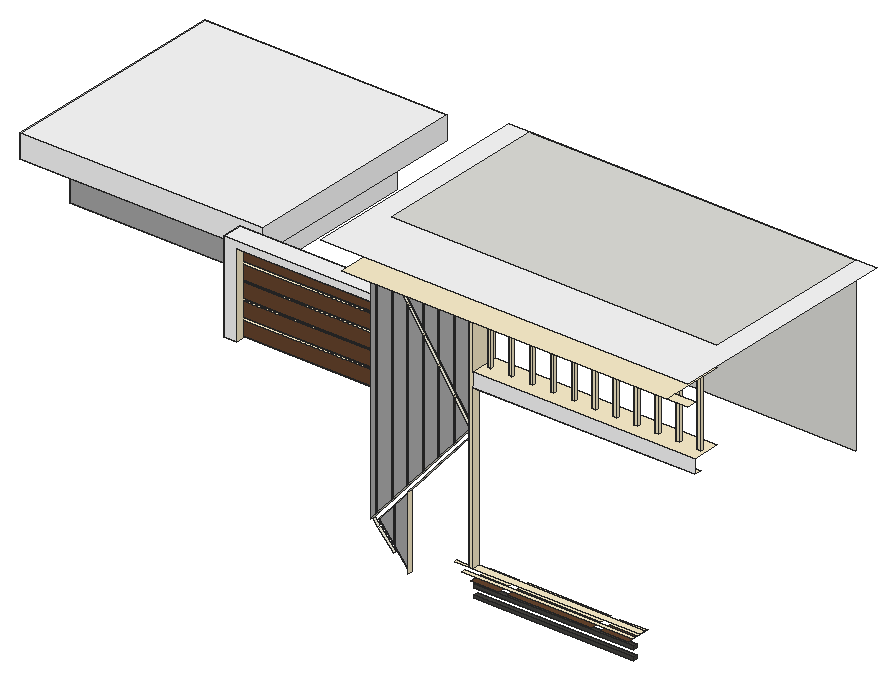
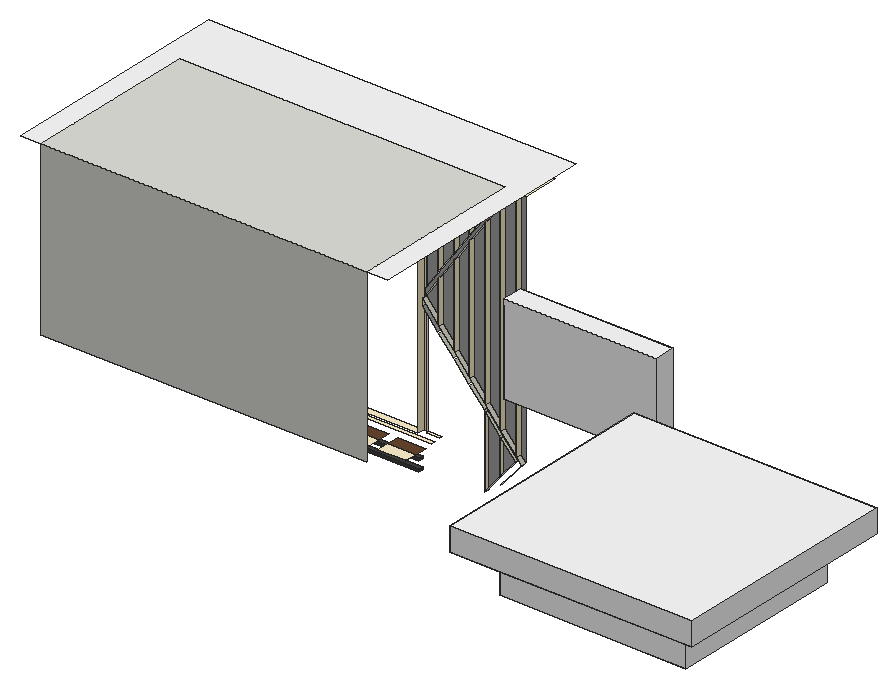
# SketchUp Ruby script. Lengths in inches.
U = 1.inch
M = Sketchup.active_model
def pt(a) = Geom::Point3d.new(a.map { |v| v * U })
def face(e, loops, mat)
  f = e.add_face(loops[0].map { |a| pt(a) })
  loops[1..].each { |l| e.add_face(l.map { |a| pt(a) }).erase! }
  f.material = f.back_material = mat if mat
  f
end
# faces: each face lists its corners as indices into pts; further lists are holes
def faces(e, pts, list, mat = nil) = list.each { |f| face(e, (f[0].is_a?(Array) ? f : [f]).map { |l| l.map { |i| pts[i] } }, mat) }
# xy, xz, yz: faces in a plane at the given z, y or x. An outline is a flat list of corners, or four numbers for a rectangle; further outlines are holes
def ring(l) = l.size == 4 ? [[l[0], l[1]], [l[2], l[1]], [l[2], l[3]], [l[0], l[3]]] : l.each_slice(2).to_a
def flat(e, list, mat, &to3) = list.each { |f| face(e, (f[0].is_a?(Array) ? f : [f]).map { |l| ring(l).map { |u, v| to3.(u, v) } }, mat) }
def xy(e, z, list, mat = nil) = flat(e, list, mat) { |x, y| [x, y, z] }
def xz(e, y, list, mat = nil) = flat(e, list, mat) { |x, z| [x, y, z] }
def yz(e, x, list, mat = nil) = flat(e, list, mat) { |y, z| [x, y, z] }
def lines(e, pts, list) = list.each { |a, b| e.add_line(pt(pts[a]), pt(pts[b])) }
# prism: a flat outline (further loops are holes) pulled along v
def prism(e, loops, v, mat = nil)
  f = face(e, loops, mat); d = Geom::Vector3d.new(v.map { |x| x * U })
  f.pushpull(f.normal.samedirection?(d) ? d.length : -d.length)
end
def box(e, o, s, mat = nil) = prism(e, [[o, [o[0] + s[0], o[1], o[2]], [o[0] + s[0], o[1] + s[1], o[2]], [o[0], o[1] + s[1], o[2]]]], [0, 0, s[2]], mat)
def at(x, y, z, deg = 0) = Geom::Transformation.translation(pt([x, y, z])) * Geom::Transformation.rotation(ORIGIN, Z_AXIS, deg.degrees)
def axes(o, x, y, z) = Geom::Transformation.new([*x, 0, *y, 0, *z, 0, *pt(o).to_a, 1])
def part(name) = M.definitions.add(name)
# library, detail: a bought-in or finely detailed component or shape, given as its bounding box
def library(name, o, s) = part(name).tap { |d| box(d.entities, o, s) }
def detail(e, o, s) = box(e.add_group.entities, o, s)
def put(e, d, t, mat = nil) = e.add_instance(d, t).tap { |i| i.material = mat if mat }
def group(e, t, mat = nil) = e.add_group.tap { |g| g.transformation = t; g.material = mat if mat }.entities
root = M.entities
M.materials.add("D01_Frost_White").color = [255, 242, 206]
M.materials.add("M00_Soft_Cloud").color = [255, 255, 255]
M.materials.add("M03_Pewter_Shine").color = [168, 168, 168]
M.materials.add("Metal_06_1K").color = [238, 236, 219]
M.materials.add("Wood_Planks_01_1K").color = [69, 67, 63]
M.materials.add("Wood_Veneer_15_1K").color = [103, 69, 45]
xy(root,235.08,[[313.01,117.13,382.01,119.15]],"Wood_Planks_01_1K")
xy(root,236.46,[[313.01,117.13,382.01,119.15]],"Wood_Planks_01_1K")
xy(root,239.33,[[313.01,117.13,382.01,119.15]],"Wood_Planks_01_1K")
xy(root,240.7,[[313.01,117.13,382.01,119.15]],"Wood_Planks_01_1K")
xy(root,242.68,[[313.01,115.54,313.02,126],[313.02,120.77,325.01,126],[329.01,120.77,365.01,126],[369.01,120.77,381.02,126]],"D01_Frost_White")
xy(root,242.68,[[313.02,115.54,325.01,120.77],[329.01,115.54,365.01,120.77],[369.01,115.54,381.02,120.77]],"Wood_Veneer_15_1K")
xy(root,245.68,[[310.01,114,384.02,115.54]],"D01_Frost_White")
xy(root,248.68,[[307.01,114,313.02,115],[315.02,114,387.02,117]],"D01_Frost_White")
xy(root,290,[[194.88,129,194.88,138,261.02,138,261.02,133.24,200.88,133.24,200.88,129],[96.73,168.8,177.62,244.72]],"D01_Frost_White")
xy(root,291,[[200.88,132.24,261.02,133.24]],"D01_Frost_White")
xy(root,297.25,[[200.88,132.24,261.02,133.24]],"D01_Frost_White")
xy(root,298.25,[[200.88,132.24,261.02,133.24]],"D01_Frost_White")
xy(root,304.5,[[200.88,132.24,261.02,133.24]],"D01_Frost_White")
xy(root,305.5,[[200.88,132.24,261.02,133.24]],"D01_Frost_White")
xy(root,308,[[96.73,168.8,177.62,244.72]],"D01_Frost_White")
xy(root,308,[[84.73,156.8,189.62,168.8],[84.73,168.8,96.73,256.72],[177.62,168.8,189.62,256.72],[96.73,244.72,177.62,256.72]],"M00_Soft_Cloud")
xy(root,311.75,[[200.88,132.24,261.02,133.24]],"D01_Frost_White")
xy(root,312.75,[[200.88,132.24,261.02,133.24]],"D01_Frost_White")
xy(root,318,[[84.73,156.8,189.62,256.72]],"M00_Soft_Cloud")
xy(root,319,[[315.02,114,387.02,117],[387.02,114,411.02,117],[200.88,132.24,261.02,133.24]],"D01_Frost_White")
xy(root,320,[[200.88,132.24,261.02,133.24]],"D01_Frost_White")
xy(root,325,[[[315.02,114,411.02,126],[316.82,119.67,318.36,120.6875]]],"D01_Frost_White")
xy(root,326,[[200.88,129,261.02,132.24]],"D01_Frost_White")
xy(root,328.95,[[194.88,129,261.02,138]],"M00_Soft_Cloud")
xy(root,355,[[270.02,99,270.02,115,272.24,115,272.24,117,272.74,117,272.74,115,275.84,115,275.84,116,277.34,116,277.34,115,278.95,115,278.95,117,279.45,117,279.45,115,285.67,115,285.67,117,286.17,117,286.17,115,292.38,115,292.38,117,292.88,117,292.88,115,299.09,115,299.09,117,299.59,117,299.59,115,305.81,115,305.81,117,306.31,117,306.31,115,313.02,115,313.02,114,315.02,114,315.02,126,411.02,126,411.02,99],[411.02,99,420.02,103.1]],"D01_Frost_White")
xy(root,356.67,[[316.82,119.67,318.36,120.6875],[325.875,119.67,327.42,120.6875],[334.93,119.67,336.47,120.6875],[343.99,119.67,345.53,120.6875],[353.05,119.67,354.59,120.6875],
  [362.11,119.67,363.65,120.6875],[371.17,119.67,372.71,120.6875],[380.23,119.67,381.77,120.6875],[389.29,119.67,390.83,120.6875],[398.34,119.67,399.88,120.6875],
  [407.4,119.67,408.94,120.6875]],"D01_Frost_White")
xy(root,364,[[270.02,126,411.02,201]])
xy(root,364,[[261.02,99,420.02,99,420.02,201,411.02,201,411.02,126,270.02,126,270.02,201,261.02,201]],"M00_Soft_Cloud")
xz(root,114,[[313.02,248.68,315.02,355]],"D01_Frost_White")
xz(root,114,[[315.02,319,411.02,325]],"M00_Soft_Cloud")
xz(root,115,[[270.02,251.83,272.24,254.41,272.24,355,270.02,355],[272.74,254.99,278.95,262.22,278.95,350.56,275.84,355,272.74,355],[279.45,262.8,285.67,270.02,285.67,340.96,279.45,349.84],[286.17,270.61,292.38,277.83,292.38,331.36,286.17,340.24],[292.88,278.41,299.09,285.64,299.09,321.76,292.88,330.64],
  [299.59,286.22,305.81,293.45,305.81,312.15,299.59,321.04],[306.31,294.03,313.02,301.84,306.31,311.44],[313.02,304.84,313.02,355,306.31,355,306.31,314.28],[305.81,314.98,305.81,355,299.59,355,299.59,323.72],[299.09,324.42,299.09,355,292.88,355,292.88,333.16],
  [292.38,333.86,292.38,355,286.17,355,286.17,342.6],[285.67,343.3,285.67,355,279.45,355,279.45,352.04],[278.95,352.74,278.95,355,277.34,355]],"M03_Pewter_Shine")
xz(root,116,[[285.67,236.55,285.67,267.27,279.45,260.1,279.45,244.15],[278.95,244.76,278.95,259.53,272.74,252.36],[313.02,301.84,313.02,304.84,306.31,314.28,305.81,314.98,299.59,323.72,299.09,324.42,292.88,333.16,292.38,333.86,286.17,342.6,285.67,343.3,279.45,352.04,278.95,352.74,277.34,355,275.84,355,278.95,350.56,279.45,349.84,285.67,340.96,286.17,340.24,292.38,331.36,292.88,330.64,299.09,321.76,299.59,321.04,305.81,312.15,306.31,311.44]],"M03_Pewter_Shine")
xz(root,117,[[286.17,235.93,286.17,267.85,285.67,267.27,285.67,236.55],[279.45,244.15,279.45,260.1,278.95,259.53,278.95,244.76],[272.24,254.41,272.74,254.99,272.74,355,272.24,355],[278.95,262.22,279.45,262.8,279.45,349.84,278.95,350.56],[285.67,270.02,286.17,270.61,286.17,340.24,285.67,340.96],
  [292.38,277.83,292.88,278.41,292.88,330.64,292.38,331.36],[299.09,285.64,299.59,286.22,299.59,321.04,299.09,321.76],[305.81,293.45,306.31,294.03,306.31,311.44,305.81,312.15],[306.31,314.28,306.31,355,305.81,355,305.81,314.98],[299.59,323.72,299.59,355,299.09,355,299.09,324.42],
  [292.88,333.16,292.88,355,292.38,355,292.38,333.86],[286.17,342.6,286.17,355,285.67,355,285.67,343.3],[279.45,352.04,279.45,355,278.95,355,278.95,352.74]],"D01_Frost_White")
xz(root,117.13,[[313.01,235.08,382.01,236.46],[313.01,239.33,382.01,240.7]],"Wood_Planks_01_1K")
xz(root,119.15,[[313.01,235.08,382.01,236.46],[313.01,239.33,382.01,240.7]],"Wood_Planks_01_1K")
xz(root,119.67,[[316.82,325,318.36,356.67],[325.875,325,327.42,356.67],[334.93,325,336.47,356.67],[343.99,325,345.53,356.67],[353.05,325,354.59,356.67],
  [362.11,325,363.65,356.67],[371.17,325,372.71,356.67],[380.23,325,381.77,356.67],[389.29,325,390.83,356.67],[398.34,325,399.88,356.67],
  [407.4,325,408.94,356.67]],"D01_Frost_White")
xz(root,120.6875,[[316.82,325,318.36,356.67],[325.875,325,327.42,356.67],[334.93,325,336.47,356.67],[343.99,325,345.53,356.67],[353.05,325,354.59,356.67],
  [362.11,325,363.65,356.67],[371.17,325,372.71,356.67],[380.23,325,381.77,356.67],[389.29,325,390.83,356.67],[398.34,325,399.88,356.67],
  [407.4,325,408.94,356.67]],"D01_Frost_White")
xz(root,129,[[194.88,290,200.88,290,200.88,326,261.02,326,261.02,328.95,194.88,328.95]],"M00_Soft_Cloud")
xz(root,132.24,[[200.88,291,261.02,297.25],[200.88,298.25,261.02,304.5],[200.88,305.5,261.02,311.75],[200.88,312.75,261.02,319],[200.88,320,261.02,326]],"Wood_Veneer_15_1K")
xz(root,133.24,[[200.88,290,261.02,291],[200.88,297.25,261.02,298.25],[200.88,304.5,261.02,305.5],[200.88,311.75,261.02,312.75],[200.88,319,261.02,320]],"D01_Frost_White")
xz(root,138,[[194.88,290,261.02,328.95]],"M00_Soft_Cloud")
xz(root,156.8,[[84.73,308,189.62,318]],"M00_Soft_Cloud")
xz(root,168.8,[[96.73,290,177.62,308]],"M03_Pewter_Shine")
xz(root,201,[[270.02,290,411.02,364]])
xz(root,244.72,[[96.73,290,177.62,308]],"M00_Soft_Cloud")
xz(root,256.72,[[84.73,308,189.62,318]],"M00_Soft_Cloud")
yz(root,84.73,[[156.8,308,256.72,318]],"M00_Soft_Cloud")
yz(root,96.73,[[168.8,290,244.72,308]],"M00_Soft_Cloud")
yz(root,177.62,[[168.8,290,244.72,308]],"M00_Soft_Cloud")
yz(root,189.62,[[156.8,308,256.72,318]],"M00_Soft_Cloud")
yz(root,194.88,[[129,290,138,328.95]],"M00_Soft_Cloud")
yz(root,200.88,[[129,290,133.24,290,133.24,291,132.24,291,132.24,297.25,133.24,297.25,133.24,298.25,132.24,298.25,132.24,304.5,133.24,304.5,133.24,305.5,132.24,305.5,132.24,311.75,133.24,311.75,133.24,312.75,132.24,312.75,132.24,319,133.24,319,133.24,320,132.24,320,132.24,326,129,326]],"D01_Frost_White")
yz(root,261.02,[[133.24,290,133.24,291,132.24,291,132.24,297.25,133.24,297.25,133.24,298.25,132.24,298.25,132.24,304.5,133.24,304.5,133.24,305.5,132.24,305.5,132.24,311.75,133.24,311.75,133.24,312.75,132.24,312.75,132.24,319,133.24,319,133.24,320,132.24,320,132.24,326,138,326,138,290]],"D01_Frost_White")
yz(root,272.24,[[115,254.41,117,355]],"D01_Frost_White")
yz(root,272.74,[[115,254.99,117,355]],"D01_Frost_White")
yz(root,278.95,[[116,244.76,117,259.53],[115,262.22,117,350.56],[115,352.74,117,355]],"D01_Frost_White")
yz(root,279.45,[[116,244.15,117,260.1],[115,262.8,117,349.84],[115,352.04,117,355]],"D01_Frost_White")
yz(root,285.67,[[116,236.55,117,267.27],[115,270.02,117,340.96],[115,343.3,117,355]],"D01_Frost_White")
yz(root,286.17,[[115,235.93,117,267.85],[115,270.61,117,340.24],[115,342.6,117,355]],"D01_Frost_White")
yz(root,292.38,[[115,277.83,117,331.36],[115,333.86,117,355]],"D01_Frost_White")
yz(root,292.88,[[115,278.41,117,330.64],[115,333.16,117,355]],"D01_Frost_White")
yz(root,299.09,[[115,285.64,117,321.76],[115,324.42,117,355]],"D01_Frost_White")
yz(root,299.59,[[115,286.22,117,321.04],[115,323.72,117,355]],"D01_Frost_White")
yz(root,305.81,[[115,293.45,117,312.15],[115,314.98,117,355]],"D01_Frost_White")
yz(root,306.31,[[115,294.03,117,311.44],[115,314.28,117,355]],"D01_Frost_White")
yz(root,313.02,[[114,248.68,115,298.84],[114,298.84,114,355,115,355,115,304.84,116,304.84,116,301.84,117,301.84,117,298.84]],"D01_Frost_White")
yz(root,315.02,[[114,248.68,117,319],[114,325,126,355]],"D01_Frost_White")
yz(root,316.82,[[119.67,325,120.6875,356.67]],"D01_Frost_White")
yz(root,318.36,[[119.67,325,120.6875,356.67]],"D01_Frost_White")
yz(root,325.875,[[119.67,325,120.6875,356.67]],"D01_Frost_White")
yz(root,327.42,[[119.67,325,120.6875,356.67]],"D01_Frost_White")
yz(root,334.93,[[119.67,325,120.6875,356.67]],"D01_Frost_White")
yz(root,336.47,[[119.67,325,120.6875,356.67]],"D01_Frost_White")
yz(root,343.99,[[119.67,325,120.6875,356.67]],"D01_Frost_White")
yz(root,345.53,[[119.67,325,120.6875,356.67]],"D01_Frost_White")
yz(root,353.05,[[119.67,325,120.6875,356.67]],"D01_Frost_White")
yz(root,354.59,[[119.67,325,120.6875,356.67]],"D01_Frost_White")
yz(root,362.11,[[119.67,325,120.6875,356.67]],"D01_Frost_White")
yz(root,363.65,[[119.67,325,120.6875,356.67]],"D01_Frost_White")
yz(root,371.17,[[119.67,325,120.6875,356.67]],"D01_Frost_White")
yz(root,372.71,[[119.67,325,120.6875,356.67]],"D01_Frost_White")
yz(root,380.23,[[119.67,325,120.6875,356.67]],"D01_Frost_White")
yz(root,381.77,[[119.67,325,120.6875,356.67]],"D01_Frost_White")
yz(root,382.01,[[117.13,235.08,119.15,236.46],[117.13,239.33,119.15,240.7]],"Wood_Planks_01_1K")
yz(root,389.29,[[119.67,325,120.6875,356.67]],"D01_Frost_White")
yz(root,390.83,[[119.67,325,120.6875,356.67]],"D01_Frost_White")
yz(root,398.34,[[119.67,325,120.6875,356.67]],"D01_Frost_White")
yz(root,399.88,[[119.67,325,120.6875,356.67]],"D01_Frost_White")
yz(root,407.4,[[119.67,325,120.6875,356.67]],"D01_Frost_White")
yz(root,408.94,[[119.67,325,120.6875,356.67]],"D01_Frost_White")
p = [[285.67,116,236.55],[279.45,116,244.15],[279.45,117,244.15],[285.67,117,236.55],[272.74,116,248.57],[278.95,116,241.12],
  [278.95,117,241.12],[272.74,117,248.57],[278.95,116,244.76],[272.74,116,252.36],[272.74,117,252.36],[278.95,117,244.76],
  [270.02,116,251.83],[272.24,116,249.17],[272.24,117,249.17],[270.02,117,251.83],[272.24,115,254.41],[270.02,115,251.83],
  [272.24,117,254.41],[278.95,116,259.53],[278.95,117,259.53],[278.95,115,262.22],[272.74,115,254.99],[272.74,117,254.99],
  [278.95,117,262.22],[279.45,116,260.1],[285.67,116,267.27],[285.67,117,267.27],[279.45,117,260.1],[285.67,115,270.02],
  [279.45,115,262.8],[279.45,117,262.8],[285.67,117,270.02],[286.17,115,267.85],[292.38,115,275.02],[292.38,117,275.02],
  [286.17,117,267.85],[292.38,115,277.83],[286.17,115,270.61],[286.17,117,270.61],[292.38,117,277.83],[292.88,115,275.6],
  [299.09,115,282.77],[299.09,117,282.77],[292.88,117,275.6],[299.09,115,285.64],[292.88,115,278.41],[292.88,117,278.41],
  [299.09,117,285.64],[299.59,115,283.35],[305.81,115,290.52],[305.81,117,290.52],[299.59,117,283.35],[305.81,115,293.45],
  [299.59,115,286.22],[299.59,117,286.22],[305.81,117,293.45],[306.31,115,291.09],[313.02,115,298.84],[313.02,117,298.84],
  [306.31,117,291.09],[313.02,115,301.84],[306.31,115,294.03],[306.31,117,294.03],[313.02,117,301.84],[313.02,116,301.84],
  [306.31,115,311.44],[306.31,116,311.44],[313.02,115,304.84],[306.31,115,314.28],[306.31,116,314.28],[313.02,116,304.84],
  [305.81,117,312.15],[306.31,117,311.44],[305.81,116,312.15],[299.59,115,321.04],[305.81,115,312.15],[299.59,116,321.04],
  [306.31,117,314.28],[305.81,117,314.98],[305.81,116,314.98],[305.81,115,314.98],[299.59,115,323.72],[299.59,116,323.72],
  [299.09,117,321.76],[299.59,117,321.04],[299.09,116,321.76],[292.88,115,330.64],[299.09,115,321.76],[292.88,116,330.64],
  [299.59,117,323.72],[299.09,117,324.42],[299.09,116,324.42],[299.09,115,324.42],[292.88,115,333.16],[292.88,116,333.16],
  [292.38,117,331.36],[292.88,117,330.64],[292.38,116,331.36],[286.17,115,340.24],[292.38,115,331.36],[286.17,116,340.24],
  [292.88,117,333.16],[292.38,117,333.86],[292.38,116,333.86],[292.38,115,333.86],[286.17,115,342.6],[286.17,116,342.6],
  [285.67,117,340.96],[286.17,117,340.24],[285.67,116,340.96],[279.45,115,349.84],[285.67,115,340.96],[279.45,116,349.84],
  [286.17,117,342.6],[285.67,117,343.3],[285.67,116,343.3],[285.67,115,343.3],[279.45,115,352.04],[279.45,116,352.04],
  [278.95,117,350.56],[279.45,117,349.84],[278.95,116,350.56],[275.84,115,355],[278.95,115,350.56],[275.84,116,355],
  [279.45,117,352.04],[278.95,117,352.74],[278.95,116,352.74],[278.95,115,352.74],[277.34,115,355],[277.34,116,355]]
faces(root,p,[[0,1,2,3],[4,5,6,7],[8,9,10,11],[12,13,14,15],[16,17,12,15,18],[9,19,20,10],[21,22,23,24],[25,26,27,28],
  [29,30,31,32],[33,34,35,36],[37,38,39,40],[41,42,43,44],[45,46,47,48],[49,50,51,52],[53,54,55,56],[61,62,63,64,65],
  [66,61,65,67],[68,69,70,71],[75,76,74,77],[81,82,83,80],[87,88,86,89],[93,94,95,92],[99,100,98,101],[105,106,107,104],
  [111,112,110,113],[117,118,119,116],[123,124,122,125],[129,130,131,128]],"Metal_06_1K")
faces(root,p,[[57,58,59,60]],"M03_Pewter_Shine")
faces(root,p,[[72,73,67,74],[78,79,80,70],[84,85,77,86],[90,91,92,83],[96,97,89,98],[102,103,104,95],[108,109,101,110],[114,115,116,107],
  [120,121,113,122],[126,127,128,119]],"D01_Frost_White")
